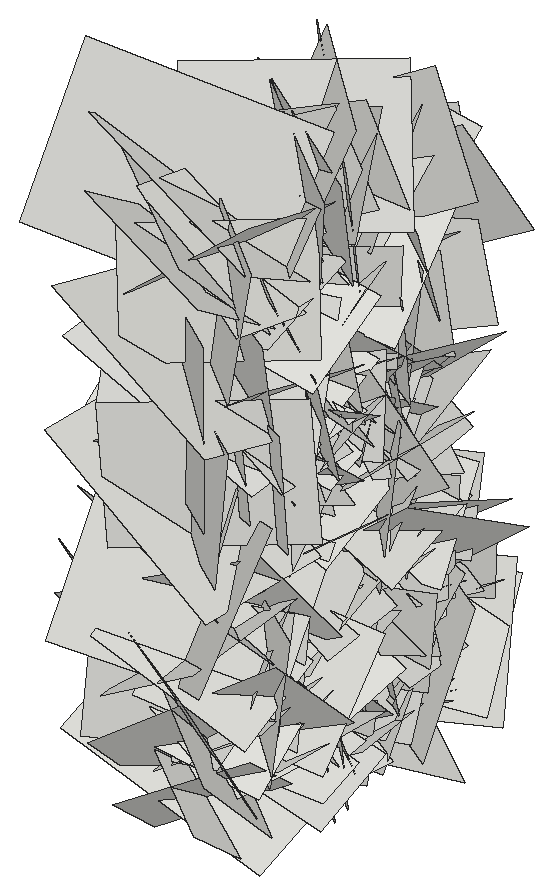
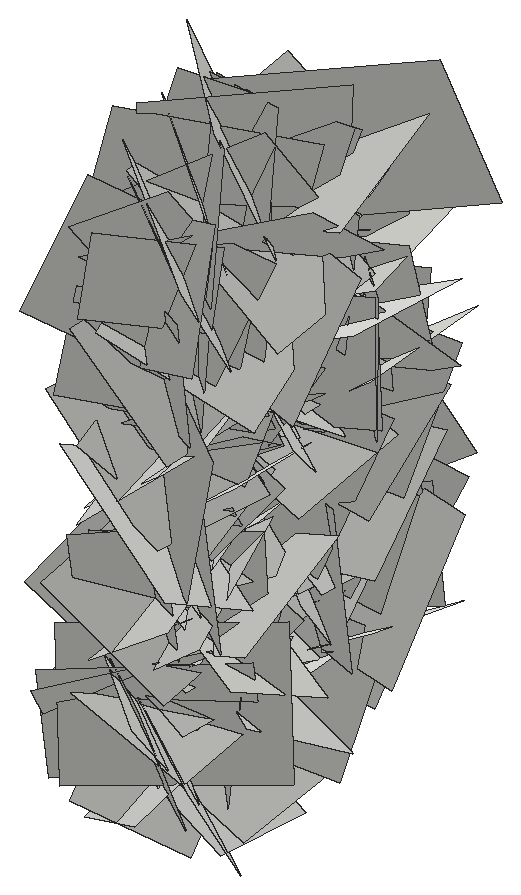
# SketchUp Ruby script. Lengths in inches.
U = 1.inch
M = Sketchup.active_model
def pt(a) = Geom::Point3d.new(a.map { |v| v * U })
def face(e, loops, mat)
  f = e.add_face(loops[0].map { |a| pt(a) })
  loops[1..].each { |l| e.add_face(l.map { |a| pt(a) }).erase! }
  f.material = f.back_material = mat if mat
  f
end
# faces: each face lists its corners as indices into pts; further lists are holes
def faces(e, pts, list, mat = nil) = list.each { |f| face(e, (f[0].is_a?(Array) ? f : [f]).map { |l| l.map { |i| pts[i] } }, mat) }
# xy, xz, yz: faces in a plane at the given z, y or x. An outline is a flat list of corners, or four numbers for a rectangle; further outlines are holes
def ring(l) = l.size == 4 ? [[l[0], l[1]], [l[2], l[1]], [l[2], l[3]], [l[0], l[3]]] : l.each_slice(2).to_a
def flat(e, list, mat, &to3) = list.each { |f| face(e, (f[0].is_a?(Array) ? f : [f]).map { |l| ring(l).map { |u, v| to3.(u, v) } }, mat) }
def xy(e, z, list, mat = nil) = flat(e, list, mat) { |x, y| [x, y, z] }
def xz(e, y, list, mat = nil) = flat(e, list, mat) { |x, z| [x, y, z] }
def yz(e, x, list, mat = nil) = flat(e, list, mat) { |y, z| [x, y, z] }
def lines(e, pts, list) = list.each { |a, b| e.add_line(pt(pts[a]), pt(pts[b])) }
# prism: a flat outline (further loops are holes) pulled along v
def prism(e, loops, v, mat = nil)
  f = face(e, loops, mat); d = Geom::Vector3d.new(v.map { |x| x * U })
  f.pushpull(f.normal.samedirection?(d) ? d.length : -d.length)
end
def box(e, o, s, mat = nil) = prism(e, [[o, [o[0] + s[0], o[1], o[2]], [o[0] + s[0], o[1] + s[1], o[2]], [o[0], o[1] + s[1], o[2]]]], [0, 0, s[2]], mat)
def at(x, y, z, deg = 0) = Geom::Transformation.translation(pt([x, y, z])) * Geom::Transformation.rotation(ORIGIN, Z_AXIS, deg.degrees)
def axes(o, x, y, z) = Geom::Transformation.new([*x, 0, *y, 0, *z, 0, *pt(o).to_a, 1])
def part(name) = M.definitions.add(name)
# library, detail: a bought-in or finely detailed component or shape, given as its bounding box
def library(name, o, s) = part(name).tap { |d| box(d.entities, o, s) }
def detail(e, o, s) = box(e.add_group.entities, o, s)
def put(e, d, t, mat = nil) = e.add_instance(d, t).tap { |i| i.material = mat if mat }
def group(e, t, mat = nil) = e.add_group.tap { |g| g.transformation = t; g.material = mat if mat }.entities
root = M.entities
c1 = part("Component\#6")
p = [[0.01,0,0],[0,3.24,4.54],[4.32,3.24,4.54],[4.33,0,0]]
faces(c1.entities,p,[[0,1,2,3]])
put(root,c1,axes([404.88,141.18,23.91],[-0.20239,-0.45291,-1.29893],[-0.24414,-1.28235,0.48098],[-1.43758,0.28153,0.10118]))
put(root,c1,axes([404.88,137.06,3.09],[-0.11239,-0.69918,1.17187],[-0.18512,1.17269,0.68387],[-1.43458,-0.09655,-0.18006]))
put(root,c1,axes([404.88,140.96,14.21],[-0.1647,-0.56811,1.02456],[-0.16232,1.03452,0.5504],[-1.23116,-0.0604,-0.20963]))
put(root,c1,axes([404.88,141.32,18.93],[0.00931,-1.12138,0.55372],[-0.26786,0.54072,1.09906],[-1.29833,-0.1196,-0.22278]))
put(root,c1,axes([404.88,142.16,14.375],[0.02255,-1.26636,-0.09652],[-0.2141,-0.09868,1.25016],[-1.3291,-0.00559,-0.20302]))
put(root,c1,axes([404.88,139.3125,6.46],[0.05297,-0.89114,0.82127],[-0.332,0.78454,0.87035],[-1.24093,-0.24794,-0.1978]))
put(root,c1,axes([404.88,148.13,7.79],[-0.13698,0.11741,-1.23467],[0.05668,-1.23967,-0.12348],[-1.31343,-0.06574,0.12344]))
put(root,c1,axes([404.88,134.59,13.6],[-0.14779,0.17555,1.29716],[0.16453,1.29751,-0.15892],[-1.37773,0.13612,-0.15813]))
put(root,c1,axes([404.88,141.11,14.91],[-0.10517,-0.78429,-0.79452],[-0.18451,-0.77703,0.78876],[-1.16892,0.19321,-0.05302]))
put(root,c1,axes([404.88,144.73,5.33],[-0.04426,-1.02294,0.56209],[-0.16257,0.56238,1.01208],[-1.2265,-0.03763,-0.15444]))
put(root,c1,axes([404.88,144.3,10.94],[-0.16969,-0.07735,1.18237],[0.06112,1.19119,0.08573],[-1.2545,0.0685,-0.15576]))
put(root,c1,axes([404.88,138.37,16.22],[-0.07456,0.76169,-0.90937],[-0.0504,-0.91204,-0.76025],[-1.25638,-0.00862,0.08446]))
put(root,c1,axes([404.88,141.48,7.17],[-0.20337,0.82379,-0.77749],[0.08888,-0.77608,-0.84298],[-1.19742,-0.19752,0.06948]))
put(root,c1,axes([404.88,139.44,14.86],[0.04621,-1.16691,0.31838],[-0.12643,0.31289,1.16311],[-1.27589,-0.07327,-0.10372]))
put(root,c1,axes([404.88,139.77,22.87],[-0.12093,1.26112,-0.05281],[0.18505,-0.03675,-1.25475],[-1.32509,-0.12022,-0.17041]))
put(root,c1,axes([404.88,146.96,20.2],[0.19126,-1.0536,-0.82739],[-0.10265,-0.84293,1.05228],[-1.41631,-0.08119,-0.188]))
put(root,c1,axes([404.88,137.94,15.45],[0.03401,0.89045,-0.73196],[-0.17038,-0.72163,-0.88493],[-1.2099,0.12665,0.10405]))
put(root,c1,axes([404.88,140.59,7.56],[0.03383,1.06332,0.50099],[-0.10932,0.50178,-1.05842],[-1.24115,-0.01522,0.10688]))
put(root,c1,axes([404.88,140.04,10.48],[0.03722,-1.27767,0.05021],[0.04996,0.05148,1.27723],[-1.35446,-0.03321,0.04849]))
put(root,c1,axes([404.88,143.08,17.68],[0.06532,-0.13436,-1.17102],[-0.13166,-1.16683,0.12734],[-1.24247,0.11658,-0.07506]))
put(root,c1,axes([404.88,141.75,2.91],[0.11729,-1.19784,-0.30033],[-0.11289,-0.30967,1.19584],[-1.30414,-0.08092,-0.13053]))
put(root,c1,axes([404.88,140.93,18.6875],[0.10901,-0.41314,-1.06231],[-0.28274,-1.04573,0.38087],[-1.17466,0.21337,-0.19026]))
put(root,c1,axes([404.88,137.64,18.89],[-0.26376,-0.64139,0.69016],[-0.02251,0.71746,0.65911],[-0.99845,0.15326,-0.19718]))
put(root,c1,axes([404.88,142.88,1.98],[-0.0351,0.64216,0.95117],[-0.00533,0.95147,-0.64254],[-1.21649,-0.02269,-0.02463]))
put(root,c1,axes([404.88,143.17,19.13],[-0.20193,0.9279,-0.28366],[-0.04691,-0.29708,-0.94209],[-1.02744,-0.16881,0.09877]))
put(root,c1,axes([404.88,137.21,11.6875],[0.11385,0.72886,-0.88593],[-0.14818,-0.87485,-0.7367],[-1.20699,0.17615,0.00688]))
put(root,c1,axes([400.91,137.29,3.46],[-0.14224,0.61257,0.15159],[0.04066,0.16261,-0.62315],[0.66768,0.1206,0.07024]))
put(root,c1,axes([404.88,138.49,4.97],[0.13436,1.04009,0.6085],[-0.04809,0.61554,-1.04268],[-1.27641,0.08629,0.10334]))
put(root,c1,axes([404.88,138.64,15.1],[0.05154,1.07135,-0.23626],[-0.10153,-0.23144,-1.06922],[-1.15847,0.06794,0.08319]))
put(root,c1,axes([404.88,142.72,8.07],[0.13823,0.05764,1.30603],[0.0986,1.30878,-0.06705],[-1.38223,0.09912,0.12583]))
put(root,c1,axes([400.91,142.82,6.12],[0.04161,-0.60559,-0.03198],[-0.13563,-0.03959,0.59276],[0.62835,0.03156,0.13006]))
put(root,c1,axes([404.88,143.54,11.83],[0.01207,0.98557,0.48784],[-0.03058,0.48797,-0.98515],[-1.16528,-0.0026,0.03091]))
put(root,c1,axes([404.88,141.07,4.77],[0.0925,1.07709,-0.24358],[-0.13853,-0.23255,-1.07513],[-1.16232,0.11343,0.10875]))
put(root,c1,axes([404.88,137.41,10.49],[-0.17918,0.96529,0.20208],[0.06958,0.21558,-0.97489],[-1.04307,-0.15144,-0.09975]))
put(root,c1,axes([404.88,139.52,8.83],[-0.01584,-0.12995,-1.07448],[-0.00128,-1.07458,0.12998],[-1.14724,0.003,0.01469]))
put(root,c1,axes([404.88,138.76,9.15],[-0.08107,-0.07376,-0.93469],[-0.12107,-0.93007,0.08274],[-0.98644,0.12021,0.06666]))
put(root,c1,axes([404.88,138.34,13.4],[-0.1901,0.66514,0.65147],[0.02496,0.66648,-0.67398],[-0.98658,-0.1113,-0.14258]))
put(root,c1,axes([404.88,141.92,3.18],[-0.02887,1.0089,0.10446],[-0.06921,0.10254,-1.00735],[-1.07292,-0.03376,0.06217]))
put(root,c1,axes([400.91,139.18,13.74],[-0.11062,-0.13563,-0.63299],[0.03095,-0.6415,0.13263],[0.6855,0.00708,-0.10814]))
put(root,c1,axes([404.88,137.89,18.97],[-0.02244,-0.79516,0.48934],[-0.22215,0.48102,0.77258],[-0.96443,-0.0923,-0.18934]))
put(root,c1,axes([404.88,137.63,3.85],[0.23328,-0.07655,1.22947],[-0.08564,1.24535,0.092],[-1.30295,-0.09556,0.21407]))
put(root,c1,axes([400.91,141.95,12.73],[-0.09992,0.55515,0.3498],[0.02862,0.35638,-0.5583],[0.69495,0.06514,0.07329]))
put(root,c1,axes([404.88,146.45,10.34],[-0.10559,0.05407,-0.92917],[-0.0532,-0.93343,-0.04894],[-0.98516,0.04461,0.10223]))
put(root,c1,axes([400.91,145.42,18.19],[-0.07853,-0.05807,0.70782],[-0.06912,0.70921,0.05136],[0.74963,0.05931,0.07889]))
put(root,c1,axes([400.91,145.36,10.15],[-0.14636,-0.64891,0.3527],[-0.01811,0.36152,0.65845],[0.78267,-0.11298,0.08119]))
put(root,c1,axes([400.91,142.6,14.22],[-0.18899,-0.6396,-0.42028],[0.00285,-0.43205,0.65638],[0.81124,-0.14749,-0.10022]))
put(root,c1,axes([400.91,139.8125,20.98],[0.02151,0.52563,-0.34386],[-0.05265,-0.34162,-0.52514],[0.66372,-0.04413,-0.03051]))
put(root,c1,axes([404.88,144.58,9.97],[-0.16827,0.58944,-0.69808],[0.0398,-0.70373,-0.60275],[-0.96765,-0.13145,0.0966]))
put(root,c1,axes([404.88,142.29,19.52],[-0.02505,0.60517,0.90894],[0.1077,0.90642,-0.60085],[-1.15246,0.07156,-0.07591]))
put(root,c1,axes([404.88,137.99,14.66],[0.08461,-0.27233,0.9902],[-0.1352,0.98287,0.28059],[-1.08015,-0.14435,0.04245]))
put(root,c1,axes([404.88,144.34,6.82],[0.01542,0.93301,-0.17325],[-0.14993,-0.1692,-0.92309],[-0.99466,0.03997,0.13646]))
put(root,c1,axes([404.88,141.25,1.55],[-0.11713,-0.0063,1.0149],[0.13715,1.01248,0.02037],[-1.06704,0.13083,-0.10878]))
put(root,c1,axes([404.88,142.2,15.72],[0.2001,0.61396,-1.10583],[0.10306,-1.12181,-0.60624],[-1.33676,0.00542,-0.21228]))
put(root,c1,axes([400.91,138.3,10.21],[-0.07821,-0.14386,0.79141],[-0.12147,0.78851,0.13265],[0.84394,0.10016,0.09244]))
put(root,c1,axes([400.91,147.58,14.43],[-0.15626,-0.88067,0.15465],[-0.14549,0.17716,0.87807],[0.93656,-0.11942,0.1622]))
put(root,c1,axes([400.91,139.99,14.29],[0.01199,-0.16574,0.68191],[-0.09091,0.67656,0.16586],[0.73829,0.086,0.00935]))
put(root,c1,axes([404.88,139.9,15.42],[-0.08068,-0.00169,-0.87701],[-0.08263,-0.87681,0.00845],[-0.92595,0.07839,0.07566]))
put(root,c1,axes([400.91,145.32,5.58],[0.01721,-0.24816,-0.73855],[-0.187,-0.7207,0.23828],[0.80443,-0.16223,0.07119]))
put(root,c1,axes([404.88,140.66,10.67],[0.05387,-0.70807,-1.02445],[0.25854,-0.99979,0.70312],[-1.29449,-0.22915,0.09779]))
put(root,c1,axes([404.88,141.11,17.69],[-0.01651,0.23078,-0.87547],[-0.12637,-0.8685,-0.22682],[-0.95135,0.11136,0.04532]))
put(root,c1,axes([400.91,138.56,10.4375],[-0.05239,0.37979,0.51244],[0.10197,0.51253,-0.37059],[0.66837,-0.04842,0.0967]))
put(root,c1,axes([404.88,149.05,6.52],[0.16475,-0.3536,-1.09271],[0.00842,-1.10231,0.35784],[-1.21738,-0.05548,-0.1454]))
put(root,c1,axes([404.88,142.09,4.39],[-0.13266,-0.06807,0.83796],[-0.05074,0.84639,0.06161],[-0.88972,-0.03812,-0.12846]))
put(root,c1,axes([404.88,136.25,6.15],[-0.02753,0.62765,0.83331],[0.11118,0.83092,-0.62258],[-1.10023,0.06826,-0.08377]))
put(root,c1,axes([400.91,141.82,12.65],[0.04235,0.31596,0.66399],[-0.14644,0.65635,-0.30401],[0.76557,0.10807,-0.09488]))
put(root,c1,axes([404.88,145.41,21.68],[-0.17174,-0.50133,-0.77339],[0.12403,-0.79008,0.48764],[-0.96905,-0.01227,0.19948]))
put(root,c1,axes([400.91,139.97,19.34],[-0.20036,-0.21311,0.82685],[-0.01235,0.84743,0.21575],[0.90502,-0.03562,0.186]))
put(root,c1,axes([404.88,135.11,11.54],[0.10699,0.00448,1.06975],[-0.01257,1.07444,-0.00338],[-1.13388,-0.01149,0.10098]))
put(root,c1,axes([400.91,141.75,2.2],[0.07408,-0.19814,0.56205],[0.01701,0.56632,0.19765],[0.63148,0.00798,-0.07126]))
put(root,c1,axes([404.88,137.79,2.1],[0.03475,-0.78477,0.75119],[0.11687,0.75006,0.77877],[-1.14558,0.05272,0.10224]))
put(root,c1,axes([400.91,139.2,5.38],[-0.02645,-0.5119,-0.36479],[0.13209,-0.36186,0.49927],[0.65307,0.05245,-0.11575]))
put(root,c1,axes([400.91,147.44,21.48],[0.11936,-0.32986,-0.48912],[-0.02265,-0.49991,0.33221],[0.62494,0.04489,0.10546]))
put(root,c1,axes([404.88,139.48,6.78],[-0.1397,0.74364,0.31774],[-0.04551,0.31504,-0.75514],[-0.85599,-0.13812,-0.01171]))
put(root,c1,axes([404.88,146.4375,4.35],[0.18242,-1.06895,0.55133],[0.10581,0.56772,1.06956],[-1.27052,-0.1062,0.16823]))
put(root,c1,axes([400.91,141.96,13.08],[0.07799,-0.57044,-0.33182],[-0.05167,-0.33766,0.56968],[0.69762,0.03877,0.07929]))
put(root,c1,axes([404.88,137.55,18.4],[0.05522,0.7917,0.38208],[-0.20111,0.38385,-0.76951],[-0.90986,-0.0368,0.19328]))
put(root,c1,axes([400.91,140.67,1.375],[0.09858,-0.02009,0.69473],[-0.09996,0.69407,0.03269],[0.72991,0.09776,-0.08935]))
put(root,c1,axes([400.91,143.63,3.63],[0.04495,-0.13338,0.65571],[0.00407,0.65706,0.13341],[0.70927,0.00468,-0.04233]))
put(root,c1,axes([400.91,139.35,17.19],[0.06054,-0.33637,0.61942],[-0.0607,0.61718,0.34043],[0.74468,0.07766,-0.02261]))
put(root,c1,axes([404.88,145.52,15.88],[0.20612,-0.51117,0.96001],[-0.04532,0.97089,0.52562],[-1.15198,-0.12966,0.1511]))
put(root,c1,axes([400.91,136.74,12.93],[0.11437,0.04247,0.59628],[0.02624,0.60507,-0.04758],[0.63311,-0.03275,-0.10574]))
put(root,c1,axes([400.91,142.73,15.75],[-0.26089,1.021,-0.12695],[-0.10549,-0.15355,-1.04195],[1.08548,0.23047,-0.13178]))
put(root,c1,axes([404.88,139.41,15.5],[-0.07329,-0.02436,0.98546],[0.16551,0.97513,0.03506],[-1.03171,0.15816,-0.06438]))
put(root,c1,axes([400.91,143.53,7.33],[-0.11895,-0.88372,0.009],[-0.0734,0.01784,0.88799],[0.93392,-0.11115,0.07094]))
put(root,c1,axes([404.88,142.07,24.73],[0.13514,0.30002,-0.93652],[-0.09595,-0.93677,-0.31242],[-1.03799,0.12565,-0.09305]))
put(root,c1,axes([400.91,138.58,20.36],[-0.30182,0.3301,1.08442],[-0.18064,1.09293,-0.37743],[1.1879,0.25007,0.21813]))
put(root,c1,axes([404.88,143.76,15.19],[-0.09057,0.86782,-0.29614],[0.1091,-0.28647,-0.86917],[-0.96584,-0.11373,-0.07041]))
put(root,c1,axes([404.88,139.77,3.95],[-0.11908,-0.78329,-0.0515],[-0.03618,-0.0471,0.79084],[-0.83129,0.11425,-0.02704]))
put(root,c1,axes([400.91,146.8125,4.55],[-0.17148,-0.83232,0.10491],[0.08015,0.09194,0.84603],[0.88562,-0.16948,-0.05625]))
put(root,c1,axes([404.88,145.52,18.22],[0.02537,0.1253,-0.85934],[-0.08829,-0.85537,-0.12704],[-0.91628,0.08589,-0.01155]))
put(root,c1,axes([404.88,143.66,16.18],[-0.1105,0.58717,-0.52568],[-0.01323,-0.53143,-0.59111],[-0.83529,-0.06926,0.0789]))
put(root,c1,axes([404.88,147.01,9.44],[0.18802,-1.10018,-0.17062],[0.06994,-0.16208,1.11371],[-1.17806,-0.18521,0.03889]))
put(root,c1,axes([400.91,143.33,2.25],[0.06381,-0.71847,0.0034],[-0.02834,0.00117,0.7205],[0.76106,0.06028,0.02655]))
put(root,c1,axes([404.88,144.05,16.5],[-0.02895,-0.76847,-0.41691],[0.01722,-0.41749,0.76847],[-0.92657,0.01625,0.02731]))
put(root,c1,axes([404.88,143.95,11.7],[0.02215,-0.88691,-0.38082],[0.08723,-0.37788,0.88459],[-1.0194,-0.05161,0.06742]))
put(root,c1,axes([400.91,147.56,10.64],[0.00206,-0.13591,-0.77504],[-0.03252,-0.77447,0.13573],[0.83344,-0.02988,0.00721]))
put(root,c1,axes([400.91,142.57,12.97],[-0.12959,-0.66136,0.5647],[0.03976,0.56572,0.67067],[0.92097,-0.11748,0.0505]))
put(root,c1,axes([404.88,141.85,18.04],[0.12661,-0.3078,1.12748],[0.24587,1.11705,0.28038],[-1.21422,0.1941,0.17434]))
put(root,c1,axes([400.91,147.06,19.23],[-0.16196,0.05609,-0.92604],[0.00217,-0.93849,-0.05718],[0.9834,0.01131,-0.15239]))
put(root,c1,axes([400.91,141.5625,11.54],[-0.13399,-0.80117,0.38482],[0.02481,0.38556,0.81039],[0.9418,-0.12414,0.0334]))
put(root,c1,axes([400.91,149.3125,5.88],[-0.15882,-0.57412,-0.80425],[-0.08368,-0.80389,0.58857],[1.04409,-0.15176,-0.07517]))
put(root,c1,axes([404.88,143.03,2.65],[0.18528,-0.93043,-0.12384],[-0.14778,-0.15031,0.9325],[-0.98392,-0.15263,-0.16338]))
put(root,c1,axes([400.91,141.35,5.69],[0.05421,0.52298,-0.48745],[0.04158,-0.49001,-0.52162],[0.75668,-0.01054,0.06359]))
put(root,c1,axes([404.88,145.65,3.28],[-0.1646,0.60158,-0.34623],[-0.0091,-0.35642,-0.61544],[-0.73568,-0.13018,0.08507]))
put(root,c1,axes([400.91,139.62,7.21],[-0.15609,-0.9187,-0.23757],[-0.00588,-0.23958,0.92989],[1.00583,-0.14396,-0.03143]))
put(root,c1,axes([400.91,143.17,8.1],[0.04482,0.75985,0.07181],[0.00358,0.07173,-0.76102],[0.80902,-0.04241,-0.00061]))
put(root,c1,axes([400.91,141.47,13.3125],[-0.15098,-0.93805,0.13539],[-0.00567,0.13771,0.94846],[1.00463,-0.1402,0.0257]))
put(root,c1,axes([404.88,139.94,18.75],[0.02341,-0.9115,0.17831],[0.09444,0.17962,0.90714],[-0.97996,-0.00447,0.09169]))
put(root,c1,axes([400.91,144.39,10.35],[-0.12238,0.87118,-0.30871],[-0.00416,-0.31157,-0.87778],[0.97971,0.1075,-0.04229]))
put(root,c1,axes([400.91,135.6875,17.375],[-0.11773,0.10526,0.9962],[-0.108,0.99592,-0.11659],[1.05635,0.11356,0.09911]))
put(root,c1,axes([400.91,136.7,5.12],[0.11008,0.58852,-0.4619],[-0.03608,-0.46213,-0.59646],[0.7922,-0.10282,0.03702]))
put(root,c1,axes([404.88,147.32,10.4375],[0.06119,-0.47987,-0.75245],[0.01649,-0.75336,0.48165],[-0.94584,-0.04418,-0.04028]))
put(root,c1,axes([400.91,147.32,10.4375],[-0.06119,-0.47987,-0.75245],[-0.01649,-0.75336,0.48165],[0.94584,-0.04418,-0.04028]))
put(root,c1,axes([404.88,136.7,5.12],[-0.11008,0.58852,-0.4619],[0.03608,-0.46213,-0.59646],[-0.7922,-0.10282,0.03702]))
put(root,c1,axes([404.88,135.6875,17.375],[0.11773,0.10526,0.9962],[0.108,0.99592,-0.11659],[-1.05635,0.11356,0.09911]))
put(root,c1,axes([404.88,144.39,10.35],[0.12238,0.87118,-0.30871],[0.00416,-0.31157,-0.87778],[-0.97971,0.1075,-0.04229]))
put(root,c1,axes([400.91,139.94,18.75],[-0.02341,-0.9115,0.17831],[-0.09444,0.17962,0.90714],[0.97996,-0.00447,0.09169]))
put(root,c1,axes([404.88,141.47,13.3125],[0.15098,-0.93805,0.13539],[0.00567,0.13771,0.94846],[-1.00463,-0.1402,0.0257]))
put(root,c1,axes([404.88,143.17,8.1],[-0.04482,0.75985,0.07181],[-0.00358,0.07173,-0.76102],[-0.80902,-0.04241,-0.00061]))
put(root,c1,axes([404.88,139.62,7.21],[0.15609,-0.9187,-0.23757],[0.00588,-0.23958,0.92989],[-1.00583,-0.14396,-0.03143]))
put(root,c1,axes([400.91,145.65,3.28],[0.1646,0.60158,-0.34623],[0.0091,-0.35642,-0.61544],[0.73568,-0.13018,0.08507]))
put(root,c1,axes([404.88,141.35,5.69],[-0.05421,0.52298,-0.48745],[-0.04158,-0.49001,-0.52162],[-0.75668,-0.01054,0.06359]))
put(root,c1,axes([400.91,143.03,2.65],[-0.18528,-0.93043,-0.12384],[0.14778,-0.15031,0.9325],[0.98392,-0.15263,-0.16338]))
put(root,c1,axes([404.88,149.3125,5.88],[0.15882,-0.57412,-0.80425],[0.08368,-0.80389,0.58857],[-1.04409,-0.15176,-0.07517]))
put(root,c1,axes([404.88,141.5625,11.54],[0.13399,-0.80117,0.38482],[-0.02481,0.38556,0.81039],[-0.9418,-0.12414,0.0334]))
put(root,c1,axes([404.88,147.06,19.23],[0.16196,0.05609,-0.92604],[-0.00217,-0.93849,-0.05718],[-0.9834,0.01131,-0.15239]))
put(root,c1,axes([400.91,141.85,18.04],[-0.12661,-0.3078,1.12748],[-0.24587,1.11705,0.28038],[1.21422,0.1941,0.17434]))
put(root,c1,axes([404.88,142.57,12.97],[0.12959,-0.66136,0.5647],[-0.03976,0.56572,0.67067],[-0.92097,-0.11748,0.0505]))
put(root,c1,axes([404.88,147.56,10.64],[-0.00206,-0.13591,-0.77504],[0.03252,-0.77447,0.13573],[-0.83344,-0.02988,0.00721]))
put(root,c1,axes([400.91,143.95,11.7],[-0.02215,-0.88691,-0.38082],[-0.08723,-0.37788,0.88459],[1.0194,-0.05161,0.06742]))
put(root,c1,axes([400.91,144.05,16.5],[0.02895,-0.76847,-0.41691],[-0.01722,-0.41749,0.76847],[0.92657,0.01625,0.02731]))
put(root,c1,axes([404.88,143.33,2.25],[-0.06381,-0.71847,0.0034],[0.02834,0.00117,0.7205],[-0.76106,0.06028,0.02655]))
put(root,c1,axes([400.91,147.01,9.44],[-0.18802,-1.10018,-0.17062],[-0.06994,-0.16208,1.11371],[1.17806,-0.18521,0.03889]))
put(root,c1,axes([400.91,143.66,16.18],[0.1105,0.58717,-0.52568],[0.01323,-0.53143,-0.59111],[0.83529,-0.06926,0.0789]))
put(root,c1,axes([400.91,145.52,18.22],[-0.02537,0.1253,-0.85934],[0.08829,-0.85537,-0.12704],[0.91628,0.08589,-0.01155]))
put(root,c1,axes([404.88,146.8125,4.55],[0.17148,-0.83232,0.10491],[-0.08015,0.09194,0.84603],[-0.88562,-0.16948,-0.05625]))
put(root,c1,axes([400.91,139.77,3.95],[0.11908,-0.78329,-0.0515],[0.03618,-0.0471,0.79084],[0.83129,0.11425,-0.02704]))
put(root,c1,axes([400.91,143.76,15.19],[0.09057,0.86782,-0.29614],[-0.1091,-0.28647,-0.86917],[0.96584,-0.11373,-0.07041]))
put(root,c1,axes([404.88,138.58,20.36],[0.30182,0.3301,1.08442],[0.18064,1.09293,-0.37743],[-1.1879,0.25007,0.21813]))
put(root,c1,axes([400.91,142.07,24.73],[-0.13514,0.30002,-0.93652],[0.09595,-0.93677,-0.31242],[1.03799,0.12565,-0.09305]))
put(root,c1,axes([404.88,143.53,7.33],[0.11895,-0.88372,0.009],[0.0734,0.01784,0.88799],[-0.93392,-0.11115,0.07094]))
put(root,c1,axes([400.91,139.41,15.5],[0.07329,-0.02436,0.98546],[-0.16551,0.97513,0.03506],[1.03171,0.15816,-0.06438]))
put(root,c1,axes([404.88,142.73,15.75],[0.26089,1.021,-0.12695],[0.10549,-0.15355,-1.04195],[-1.08548,0.23047,-0.13178]))
put(root,c1,axes([404.88,136.74,12.93],[-0.11437,0.04247,0.59628],[-0.02624,0.60507,-0.04758],[-0.63311,-0.03275,-0.10574]))
put(root,c1,axes([400.91,145.52,15.88],[-0.20612,-0.51117,0.96001],[0.04532,0.97089,0.52562],[1.15198,-0.12966,0.1511]))
put(root,c1,axes([404.88,139.35,17.19],[-0.06054,-0.33637,0.61942],[0.0607,0.61718,0.34043],[-0.74468,0.07766,-0.02261]))
put(root,c1,axes([404.88,143.63,3.63],[-0.04495,-0.13338,0.65571],[-0.00407,0.65706,0.13341],[-0.70927,0.00468,-0.04233]))
put(root,c1,axes([404.88,140.67,1.375],[-0.09858,-0.02009,0.69473],[0.09996,0.69407,0.03269],[-0.72991,0.09776,-0.08935]))
put(root,c1,axes([400.91,137.55,18.4],[-0.05522,0.7917,0.38208],[0.20111,0.38385,-0.76951],[0.90986,-0.0368,0.19328]))
put(root,c1,axes([404.88,141.96,13.08],[-0.07799,-0.57044,-0.33182],[0.05167,-0.33766,0.56968],[-0.69762,0.03877,0.07929]))
put(root,c1,axes([400.91,146.4375,4.35],[-0.18242,-1.06895,0.55133],[-0.10581,0.56772,1.06956],[1.27052,-0.1062,0.16823]))
put(root,c1,axes([400.91,139.48,6.78],[0.1397,0.74364,0.31774],[0.04551,0.31504,-0.75514],[0.85599,-0.13812,-0.01171]))
put(root,c1,axes([404.88,147.44,21.48],[-0.11936,-0.32986,-0.48912],[0.02265,-0.49991,0.33221],[-0.62494,0.04489,0.10546]))
put(root,c1,axes([404.88,139.2,5.38],[0.02645,-0.5119,-0.36479],[-0.13209,-0.36186,0.49927],[-0.65307,0.05245,-0.11575]))
put(root,c1,axes([400.91,137.79,2.1],[-0.03475,-0.78477,0.75119],[-0.11687,0.75006,0.77877],[1.14558,0.05272,0.10224]))
put(root,c1,axes([404.88,141.75,2.2],[-0.07408,-0.19814,0.56205],[-0.01701,0.56632,0.19765],[-0.63148,0.00798,-0.07126]))
put(root,c1,axes([400.91,135.11,11.54],[-0.10699,0.00448,1.06975],[0.01257,1.07444,-0.00338],[1.13388,-0.01149,0.10098]))
put(root,c1,axes([404.88,139.97,19.34],[0.20036,-0.21311,0.82685],[0.01235,0.84743,0.21575],[-0.90502,-0.03562,0.186]))
put(root,c1,axes([400.91,145.41,21.68],[0.17174,-0.50133,-0.77339],[-0.12403,-0.79008,0.48764],[0.96905,-0.01227,0.19948]))
put(root,c1,axes([404.88,141.82,12.65],[-0.04235,0.31596,0.66399],[0.14644,0.65635,-0.30401],[-0.76557,0.10807,-0.09488]))
put(root,c1,axes([400.91,136.25,6.15],[0.02753,0.62765,0.83331],[-0.11118,0.83092,-0.62258],[1.10023,0.06826,-0.08377]))
put(root,c1,axes([400.91,142.09,4.39],[0.13266,-0.06807,0.83796],[0.05074,0.84639,0.06161],[0.88972,-0.03812,-0.12846]))
put(root,c1,axes([400.91,149.05,6.52],[-0.16475,-0.3536,-1.09271],[-0.00842,-1.10231,0.35784],[1.21738,-0.05548,-0.1454]))
put(root,c1,axes([404.88,138.56,10.4375],[0.05239,0.37979,0.51244],[-0.10197,0.51253,-0.37059],[-0.66837,-0.04842,0.0967]))
put(root,c1,axes([400.91,141.11,17.69],[0.01651,0.23078,-0.87547],[0.12637,-0.8685,-0.22682],[0.95135,0.11136,0.04532]))
put(root,c1,axes([400.91,140.66,10.67],[-0.05387,-0.70807,-1.02445],[-0.25854,-0.99979,0.70312],[1.29449,-0.22915,0.09779]))
put(root,c1,axes([404.88,145.32,5.58],[-0.01721,-0.24816,-0.73855],[0.187,-0.7207,0.23828],[-0.80443,-0.16223,0.07119]))
put(root,c1,axes([400.91,139.9,15.42],[0.08068,-0.00169,-0.87701],[0.08263,-0.87681,0.00845],[0.92595,0.07839,0.07566]))
